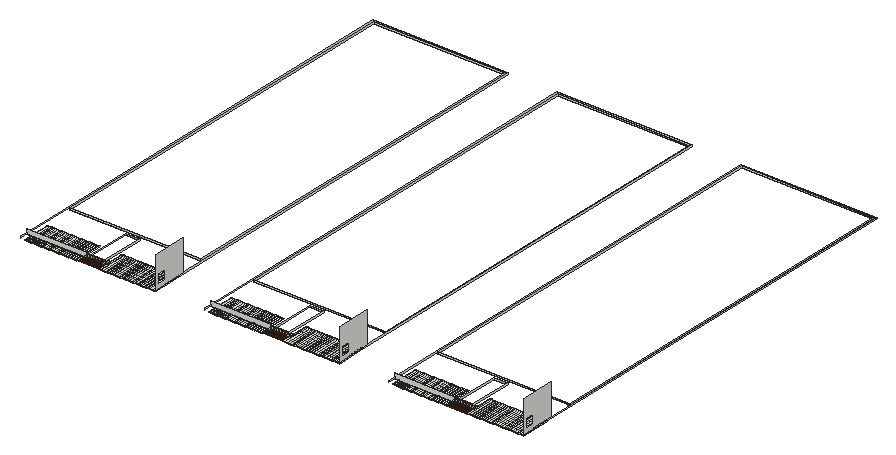
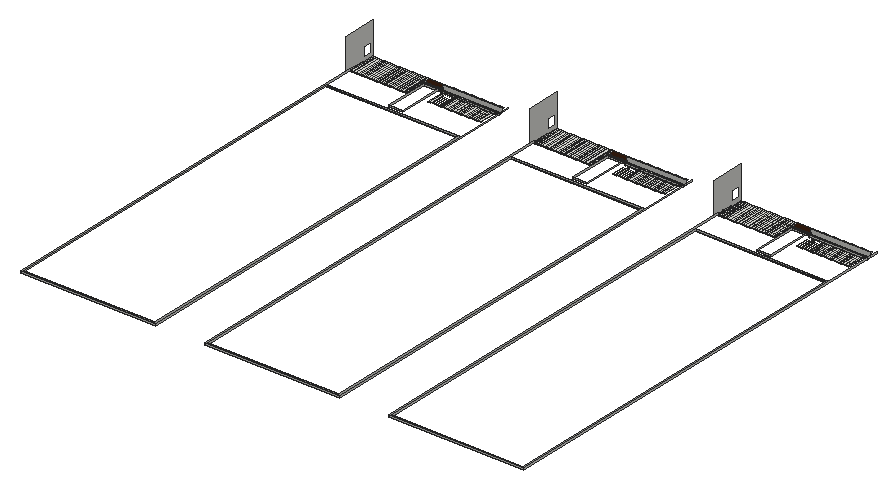
# SketchUp Ruby script. Lengths in inches.
U = 1.inch
M = Sketchup.active_model
def pt(a) = Geom::Point3d.new(a.map { |v| v * U })
def face(e, loops, mat)
  f = e.add_face(loops[0].map { |a| pt(a) })
  loops[1..].each { |l| e.add_face(l.map { |a| pt(a) }).erase! }
  f.material = f.back_material = mat if mat
  f
end
# faces: each face lists its corners as indices into pts; further lists are holes
def faces(e, pts, list, mat = nil) = list.each { |f| face(e, (f[0].is_a?(Array) ? f : [f]).map { |l| l.map { |i| pts[i] } }, mat) }
# xy, xz, yz: faces in a plane at the given z, y or x. An outline is a flat list of corners, or four numbers for a rectangle; further outlines are holes
def ring(l) = l.size == 4 ? [[l[0], l[1]], [l[2], l[1]], [l[2], l[3]], [l[0], l[3]]] : l.each_slice(2).to_a
def flat(e, list, mat, &to3) = list.each { |f| face(e, (f[0].is_a?(Array) ? f : [f]).map { |l| ring(l).map { |u, v| to3.(u, v) } }, mat) }
def xy(e, z, list, mat = nil) = flat(e, list, mat) { |x, y| [x, y, z] }
def xz(e, y, list, mat = nil) = flat(e, list, mat) { |x, z| [x, y, z] }
def yz(e, x, list, mat = nil) = flat(e, list, mat) { |y, z| [x, y, z] }
def lines(e, pts, list) = list.each { |a, b| e.add_line(pt(pts[a]), pt(pts[b])) }
# prism: a flat outline (further loops are holes) pulled along v
def prism(e, loops, v, mat = nil)
  f = face(e, loops, mat); d = Geom::Vector3d.new(v.map { |x| x * U })
  f.pushpull(f.normal.samedirection?(d) ? d.length : -d.length)
end
def box(e, o, s, mat = nil) = prism(e, [[o, [o[0] + s[0], o[1], o[2]], [o[0] + s[0], o[1] + s[1], o[2]], [o[0], o[1] + s[1], o[2]]]], [0, 0, s[2]], mat)
def at(x, y, z, deg = 0) = Geom::Transformation.translation(pt([x, y, z])) * Geom::Transformation.rotation(ORIGIN, Z_AXIS, deg.degrees)
def axes(o, x, y, z) = Geom::Transformation.new([*x, 0, *y, 0, *z, 0, *pt(o).to_a, 1])
def part(name) = M.definitions.add(name)
# library, detail: a bought-in or finely detailed component or shape, given as its bounding box
def library(name, o, s) = part(name).tap { |d| box(d.entities, o, s) }
def detail(e, o, s) = box(e.add_group.entities, o, s)
def put(e, d, t, mat = nil) = e.add_instance(d, t).tap { |i| i.material = mat if mat }
def group(e, t, mat = nil) = e.add_group.tap { |g| g.transformation = t; g.material = mat if mat }.entities
root = M.entities
M.materials.add("[Wood Veneer 01]").color = [51, 28, 15]
xy(root,505.1875,[[253.94,246.64,259.43,361.27],[987.51,246.64,993,361.27],[1721.07,246.64,1726.56,361.27]])
xy(root,505.3125,[[100.18,246.64,109.94,361.27],[109.94,246.64,115.43,361.27],[115.43,246.64,117.94,361.27],[117.94,246.64,123.43,361.27],[123.43,246.64,125.94,361.27],
  [125.94,246.64,131.43,361.27],[131.43,246.64,133.94,361.27],[133.94,246.64,139.43,361.27],[139.43,246.64,141.94,361.27],[141.94,246.64,147.43,361.27],
  [147.43,246.64,149.94,361.27],[149.94,246.64,155.43,361.27],[155.43,246.64,157.94,361.27],[157.94,246.64,163.43,361.27],[163.43,246.64,165.94,361.27],
  [165.94,246.64,171.43,361.27],[171.43,246.64,173.94,361.27],[173.94,246.64,179.43,361.27],[179.43,246.64,181.94,361.27],[181.94,246.64,187.43,361.27],
  [187.43,246.64,189.94,361.27],[189.94,246.64,195.43,361.27],[195.43,246.64,197.94,361.27],[197.94,246.64,203.43,361.27],[203.43,246.64,205.94,361.27],
  [205.94,246.64,211.43,361.27],[211.43,246.64,213.94,361.27],[213.94,246.64,219.43,361.27],[219.43,246.64,221.94,361.27],[221.94,246.64,227.43,361.27],
  [227.43,246.64,229.94,361.27],[229.94,246.64,235.43,361.27],[235.43,246.64,237.94,361.27],[237.94,246.64,243.43,361.27],[243.43,246.64,245.94,361.27],
  [245.94,246.64,251.43,361.27],[251.43,246.64,253.94,361.27],[259.43,246.64,261.94,361.27],[267.43,246.64,269.94,361.27],[275.43,246.64,277.94,361.27],
  [283.43,246.64,285.94,361.27],[291.43,246.64,293.94,361.27],[299.43,246.64,301.94,361.27],[307.43,246.64,309.94,361.27],[396.57,246.64,403.28,361.27],
  [403.28,246.64,405.07,361.27],[405.07,246.64,411.78,361.27],[411.78,246.64,413.57,361.27],[413.57,246.64,420.28,361.27],[420.28,246.64,422.07,361.27],
  [422.07,246.64,428.78,361.27],[428.78,246.64,430.57,361.27],[430.57,246.64,437.28,361.27],[437.28,246.64,439.07,361.27],[439.07,246.64,445.78,361.27],
  [445.78,246.64,447.57,361.27],[447.57,246.64,454.28,361.27],[454.28,246.64,456.07,361.27],[456.07,246.64,462.78,361.27],[462.78,246.64,464.57,361.27],
  [464.57,246.64,471.28,361.27],[471.28,246.64,473.07,361.27],[473.07,246.64,479.78,361.27],[479.78,246.64,481.57,361.27],[481.57,246.64,488.28,361.27],
  [488.28,246.64,490.07,361.27],[490.07,246.64,496.78,361.27],[496.78,246.64,498.57,361.27],[498.57,246.64,505.28,361.27],[505.28,246.64,507.07,361.27],
  [507.07,246.64,513.78,361.27],[513.78,246.64,515.57,361.27],[515.57,246.64,522.28,361.27],[522.28,246.64,524.07,361.27],[524.07,246.64,530.78,361.27],
  [530.78,246.64,532.57,361.27],[532.57,246.64,539.28,361.27],[539.28,246.64,541.07,361.27],[541.07,246.64,547.78,361.27],[547.78,246.64,549.57,361.27],
  [549.57,246.64,556.28,361.27],[556.28,246.64,558.07,361.27],[558.07,246.64,564.78,361.27],[564.78,246.64,566.57,361.27],[566.57,246.64,573.28,361.27],
  [573.28,246.64,575.07,361.27],[575.07,246.64,581.78,361.27],[581.78,246.64,583.57,361.27],[583.57,246.64,590.28,361.27],[590.28,246.64,592.07,361.27],
  [592.07,246.64,598.78,361.27],[598.78,246.64,600.57,361.27],[600.57,246.64,607.28,361.27],[607.28,246.64,609.07,361.27],[609.07,246.64,615.78,361.27],
  [615.78,246.64,617.57,361.27],[617.57,246.64,622,361.27],[833.74,246.64,843.51,361.27],[843.51,246.64,849,361.27],[849,246.64,851.51,361.27],
  [851.51,246.64,857,361.27],[857,246.64,859.51,361.27],[859.51,246.64,865,361.27],[865,246.64,867.51,361.27],[867.51,246.64,873,361.27],
  [873,246.64,875.51,361.27],[875.51,246.64,881,361.27],[881,246.64,883.51,361.27],[883.51,246.64,889,361.27],[889,246.64,891.51,361.27],
  [891.51,246.64,897,361.27],[897,246.64,899.51,361.27],[899.51,246.64,905,361.27],[905,246.64,907.51,361.27],[907.51,246.64,913,361.27],
  [913,246.64,915.51,361.27],[915.51,246.64,921,361.27],[921,246.64,923.51,361.27],[923.51,246.64,929,361.27],[929,246.64,931.51,361.27],
  [931.51,246.64,937,361.27],[937,246.64,939.51,361.27],[939.51,246.64,945,361.27],[945,246.64,947.51,361.27],[947.51,246.64,953,361.27],
  [953,246.64,955.51,361.27],[955.51,246.64,961,361.27],[961,246.64,963.51,361.27],[963.51,246.64,969,361.27],[969,246.64,971.51,361.27],
  [971.51,246.64,977,361.27],[977,246.64,979.51,361.27],[979.51,246.64,985,361.27],[985,246.64,987.51,361.27],[993,246.64,995.51,361.27],
  [1001,246.64,1003.51,361.27],[1009,246.64,1011.51,361.27],[1017,246.64,1019.51,361.27],[1025,246.64,1027.51,361.27],[1033,246.64,1035.51,361.27],
  [1041,246.64,1043.51,361.27],[1130.14,246.64,1136.84,361.27],[1136.84,246.64,1138.64,361.27],[1138.64,246.64,1145.34,361.27],[1145.34,246.64,1147.14,361.27],
  [1147.14,246.64,1153.84,361.27],[1153.84,246.64,1155.64,361.27],[1155.64,246.64,1162.34,361.27],[1162.34,246.64,1164.14,361.27],[1164.14,246.64,1170.84,361.27],
  [1170.84,246.64,1172.64,361.27],[1172.64,246.64,1179.34,361.27],[1179.34,246.64,1181.14,361.27],[1181.14,246.64,1187.84,361.27],[1187.84,246.64,1189.64,361.27],
  [1189.64,246.64,1196.34,361.27],[1196.34,246.64,1198.14,361.27],[1198.14,246.64,1204.84,361.27],[1204.84,246.64,1206.64,361.27],[1206.64,246.64,1213.34,361.27],
  [1213.34,246.64,1215.14,361.27],[1215.14,246.64,1221.84,361.27],[1221.84,246.64,1223.64,361.27],[1223.64,246.64,1230.34,361.27],[1230.34,246.64,1232.14,361.27],
  [1232.14,246.64,1238.84,361.27],[1238.84,246.64,1240.64,361.27],[1240.64,246.64,1247.34,361.27],[1247.34,246.64,1249.14,361.27],[1249.14,246.64,1255.84,361.27],
  [1255.84,246.64,1257.64,361.27],[1257.64,246.64,1264.34,361.27],[1264.34,246.64,1266.14,361.27],[1266.14,246.64,1272.84,361.27],[1272.84,246.64,1274.64,361.27],
  [1274.64,246.64,1281.34,361.27],[1281.34,246.64,1283.14,361.27],[1283.14,246.64,1289.84,361.27],[1289.84,246.64,1291.64,361.27],[1291.64,246.64,1298.34,361.27],
  [1298.34,246.64,1300.14,361.27],[1300.14,246.64,1306.84,361.27],[1306.84,246.64,1308.64,361.27],[1308.64,246.64,1315.34,361.27],[1315.34,246.64,1317.14,361.27],
  [1317.14,246.64,1323.84,361.27],[1323.84,246.64,1325.64,361.27],[1325.64,246.64,1332.34,361.27],[1332.34,246.64,1334.14,361.27],[1334.14,246.64,1340.84,361.27],
  [1340.84,246.64,1342.64,361.27],[1342.64,246.64,1349.34,361.27],[1349.34,246.64,1351.14,361.27],[1351.14,246.64,1355.5625,361.27],[1567.3,246.64,1577.07,361.27],
  [1577.07,246.64,1582.56,361.27],[1582.56,246.64,1585.07,361.27],[1585.07,246.64,1590.56,361.27],[1590.56,246.64,1593.07,361.27],[1593.07,246.64,1598.56,361.27],
  [1598.56,246.64,1601.07,361.27],[1601.07,246.64,1606.56,361.27],[1606.56,246.64,1609.07,361.27],[1609.07,246.64,1614.56,361.27],[1614.56,246.64,1617.07,361.27],
  [1617.07,246.64,1622.56,361.27],[1622.56,246.64,1625.07,361.27],[1625.07,246.64,1630.56,361.27],[1630.56,246.64,1633.07,361.27],[1633.07,246.64,1638.56,361.27],
  [1638.56,246.64,1641.07,361.27],[1641.07,246.64,1646.56,361.27],[1646.56,246.64,1649.07,361.27],[1649.07,246.64,1654.56,361.27],[1654.56,246.64,1657.07,361.27],
  [1657.07,246.64,1662.56,361.27],[1662.56,246.64,1665.07,361.27],[1665.07,246.64,1670.56,361.27],[1670.56,246.64,1673.07,361.27],[1673.07,246.64,1678.56,361.27],
  [1678.56,246.64,1681.07,361.27],[1681.07,246.64,1686.56,361.27],[1686.56,246.64,1689.07,361.27],[1689.07,246.64,1694.56,361.27],[1694.56,246.64,1697.07,361.27],
  [1697.07,246.64,1702.56,361.27],[1702.56,246.64,1705.07,361.27],[1705.07,246.64,1710.56,361.27],[1710.56,246.64,1713.07,361.27],[1713.07,246.64,1718.56,361.27],
  [1718.56,246.64,1721.07,361.27],[1726.56,246.64,1729.07,361.27],[1734.56,246.64,1737.07,361.27],[1742.56,246.64,1745.07,361.27],[1750.56,246.64,1753.07,361.27],
  [1758.56,246.64,1761.07,361.27],[1766.56,246.64,1769.07,361.27],[1774.56,246.64,1777.07,361.27],[1863.7,246.64,1870.4,361.27],[1870.4,246.64,1872.2,361.27],
  [1872.2,246.64,1878.9,361.27],[1878.9,246.64,1880.7,361.27],[1880.7,246.64,1887.4,361.27],[1887.4,246.64,1889.2,361.27],[1889.2,246.64,1895.9,361.27],
  [1895.9,246.64,1897.7,361.27],[1897.7,246.64,1904.4,361.27],[1904.4,246.64,1906.2,361.27],[1906.2,246.64,1912.9,361.27],[1912.9,246.64,1914.7,361.27],
  [1914.7,246.64,1921.4,361.27],[1921.4,246.64,1923.2,361.27],[1923.2,246.64,1929.9,361.27],[1929.9,246.64,1931.7,361.27],[1931.7,246.64,1938.4,361.27],
  [1938.4,246.64,1940.2,361.27],[1940.2,246.64,1946.9,361.27],[1946.9,246.64,1948.7,361.27],[1948.7,246.64,1955.4,361.27],[1955.4,246.64,1957.2,361.27],
  [1957.2,246.64,1963.9,361.27],[1963.9,246.64,1965.7,361.27],[1965.7,246.64,1972.4,361.27],[1972.4,246.64,1974.2,361.27],[1974.2,246.64,1980.9,361.27],
  [1980.9,246.64,1982.7,361.27],[1982.7,246.64,1989.4,361.27],[1989.4,246.64,1991.2,361.27],[1991.2,246.64,1997.9,361.27],[1997.9,246.64,1999.7,361.27],
  [1999.7,246.64,2006.4,361.27],[2006.4,246.64,2008.2,361.27],[2008.2,246.64,2014.9,361.27],[2014.9,246.64,2016.7,361.27],[2016.7,246.64,2023.4,361.27],
  [2023.4,246.64,2025.2,361.27],[2025.2,246.64,2031.9,361.27],[2031.9,246.64,2033.7,361.27],[2033.7,246.64,2040.4,361.27],[2040.4,246.64,2042.2,361.27],
  [2042.2,246.64,2048.9,361.27],[2048.9,246.64,2050.7,361.27],[2050.7,246.64,2057.4,361.27],[2057.4,246.64,2059.2,361.27],[2059.2,246.64,2065.9,361.27],
  [2065.9,246.64,2067.7,361.27],[2067.7,246.64,2074.4,361.27],[2074.4,246.64,2076.2,361.27],[2076.2,246.64,2082.9,361.27],[2082.9,246.64,2084.7,361.27],
  [2084.7,246.64,2089.125,361.27]])
xy(root,505.3125,[[315.43,246.64,396.57,286.21],[1049,246.64,1130.14,286.21],[1782.56,246.64,1863.7,286.21]],"[Wood Veneer 01]")
xy(root,506.6875,[[106.73,254.22,113.67,256.84],[119.31,254.22,126.24,256.84],[132.68,254.22,139.62,256.84],[146.56,254.22,153.49,256.84],[840.29,254.22,847.23,256.84],
  [852.87,254.22,859.81,256.84],[866.24,254.22,873.18,256.84],[880.12,254.22,887.06,256.84],[1573.86,254.22,1580.79,256.84],[1586.43,254.22,1593.37,256.84],
  [1599.81,254.22,1606.74,256.84],[1613.68,254.22,1620.62,256.84],[106.73,256.84,113.67,263.78],[119.31,256.84,126.24,263.78],[132.68,256.84,139.62,263.78],
  [146.56,256.84,153.49,263.78],[840.29,256.84,847.23,263.78],[852.87,256.84,859.81,263.78],[866.24,256.84,873.18,263.78],[880.12,256.84,887.06,263.78],
  [1573.86,256.84,1580.79,263.78],[1586.43,256.84,1593.37,263.78],[1599.81,256.84,1606.74,263.78],[1613.68,256.84,1620.62,263.78],[90.36,483.79,614.76,488.08],
  [823.93,483.79,1348.32,488.08],[1557.49,483.79,2081.89,488.08]])
xy(root,506.8125,[[83.125,277.39,100.18,293.46],[100.18,277.39,100.18,293.46,315.43,293.46,315.43,286.21,318.81,286.21,318.81,277.39],[816.6875,277.39,833.74,293.46],[833.74,277.39,833.74,293.46,1049,293.46,1049,286.21,1052.37,286.21,1052.37,277.39],[1550.25,277.39,1567.3,293.46],
  [1567.3,277.39,1567.3,293.46,1782.56,293.46,1782.56,286.21,1785.93,286.21,1785.93,277.39]])
xz(root,246.64,[[259.43,505.1875,261.94,505.19,261.94,505.3125,259.43,505.3125],[993,505.1875,995.51,505.19,995.51,505.3125,993,505.3125],[1726.56,505.1875,1729.07,505.19,1729.07,505.3125,1726.56,505.3125],[267.43,505.21,269.94,505.3125],[1001,505.21,1003.51,505.3125],
  [1734.56,505.21,1737.07,505.3125],[275.43,505.22,277.94,505.23,277.94,505.3125,275.43,505.3125],[1009,505.22,1011.51,505.23,1011.51,505.3125,1009,505.3125],[1742.56,505.22,1745.07,505.23,1745.07,505.3125,1742.56,505.3125],[283.43,505.24,285.94,505.25,285.94,505.3125,283.43,505.3125],
  [1017,505.24,1019.51,505.25,1019.51,505.3125,1017,505.3125],[1750.56,505.24,1753.07,505.25,1753.07,505.3125,1750.56,505.3125],[291.43,505.26,293.94,505.3125],[1025,505.26,1027.51,505.3125],[1758.56,505.26,1761.07,505.3125],
  [299.43,505.28,301.94,505.3125],[1033,505.28,1035.51,505.3125],[1766.56,505.28,1769.07,505.3125],[307.43,505.29,309.94,505.3,309.94,505.3125,307.43,505.3125],[1041,505.29,1043.51,505.3,1043.51,505.3125,1041,505.3125],
  [1774.56,505.29,1777.07,505.3,1777.07,505.3125,1774.56,505.3125]])
xz(root,277.39,[[83.125,506.8125,318.81,524.9375],[816.6875,506.8125,1052.37,524.9375],[1550.25,506.8125,1785.93,524.9375]])
xz(root,286.21,[[315.43,505.3125,318.81,506.8125],[318.81,505.3125,322.23,506.8125],[322.23,505.3125,324.81,506.8125],[324.81,505.3125,328.23,506.8125],[328.23,505.3125,330.81,506.8125],
  [330.81,505.3125,334.23,506.8125],[334.23,505.3125,336.81,506.8125],[336.81,505.3125,340.23,506.8125],[340.23,505.3125,342.81,506.8125],[342.81,505.3125,346.23,506.8125],
  [346.23,505.3125,348.81,506.8125],[348.81,505.3125,352.23,506.8125],[352.23,505.3125,354.81,506.8125],[354.81,505.3125,358.23,506.8125],[358.23,505.3125,360.81,506.8125],
  [360.81,505.3125,364.23,506.8125],[364.23,505.3125,366.81,506.8125],[366.81,505.3125,370.23,506.8125],[370.23,505.3125,372.81,506.8125],[372.81,505.3125,376.23,506.8125],
  [376.23,505.3125,378.81,506.8125],[378.81,505.3125,382.23,506.8125],[382.23,505.3125,384.81,506.8125],[384.81,505.3125,388.23,506.8125],[388.23,505.3125,390.12,506.8125],
  [390.12,505.3125,393.55,506.8125],[393.55,505.3125,393.95,506.8125],[393.95,505.3125,396.57,506.8125],[1049,505.3125,1052.37,506.8125],[1052.37,505.3125,1055.8,506.8125],
  [1055.8,505.3125,1058.37,506.8125],[1058.37,505.3125,1061.8,506.8125],[1061.8,505.3125,1064.37,506.8125],[1064.37,505.3125,1067.8,506.8125],[1067.8,505.3125,1070.37,506.8125],
  [1070.37,505.3125,1073.8,506.8125],[1073.8,505.3125,1076.37,506.8125],[1076.37,505.3125,1079.8,506.8125],[1079.8,505.3125,1082.37,506.8125],[1082.37,505.3125,1085.8,506.8125],
  [1085.8,505.3125,1088.37,506.8125],[1088.37,505.3125,1091.8,506.8125],[1091.8,505.3125,1094.37,506.8125],[1094.37,505.3125,1097.8,506.8125],[1097.8,505.3125,1100.37,506.8125],
  [1100.37,505.3125,1103.8,506.8125],[1103.8,505.3125,1106.37,506.8125],[1106.37,505.3125,1109.8,506.8125],[1109.8,505.3125,1112.37,506.8125],[1112.37,505.3125,1115.8,506.8125],
  [1115.8,505.3125,1118.37,506.8125],[1118.37,505.3125,1121.8,506.8125],[1121.8,505.3125,1123.68,506.8125],[1123.68,505.3125,1127.11,506.8125],[1127.11,505.3125,1127.51,506.8125],
  [1127.51,505.3125,1130.14,506.8125],[1782.56,505.3125,1785.93,506.8125],[1785.93,505.3125,1789.36,506.8125],[1789.36,505.3125,1791.93,506.8125],[1791.93,505.3125,1795.36,506.8125],
  [1795.36,505.3125,1797.93,506.8125],[1797.93,505.3125,1801.36,506.8125],[1801.36,505.3125,1803.93,506.8125],[1803.93,505.3125,1807.36,506.8125],[1807.36,505.3125,1809.93,506.8125],
  [1809.93,505.3125,1813.36,506.8125],[1813.36,505.3125,1815.93,506.8125],[1815.93,505.3125,1819.36,506.8125],[1819.36,505.3125,1821.93,506.8125],[1821.93,505.3125,1825.36,506.8125],
  [1825.36,505.3125,1827.93,506.8125],[1827.93,505.3125,1831.36,506.8125],[1831.36,505.3125,1833.93,506.8125],[1833.93,505.3125,1837.36,506.8125],[1837.36,505.3125,1839.93,506.8125],
  [1839.93,505.3125,1843.36,506.8125],[1843.36,505.3125,1845.93,506.8125],[1845.93,505.3125,1849.36,506.8125],[1849.36,505.3125,1851.93,506.8125],[1851.93,505.3125,1855.36,506.8125],
  [1855.36,505.3125,1857.25,506.8125],[1857.25,505.3125,1860.67,506.8125],[1860.67,505.3125,1861.07,506.8125],[1861.07,505.3125,1863.7,506.8125],[315.43,506.8125,318.81,512.6875],
  [318.81,506.8125,322.23,512.6875],[322.23,506.8125,324.81,512.6875],[324.81,506.8125,328.23,512.6875],[328.23,506.8125,330.81,512.6875],[330.81,506.8125,334.23,512.6875],
  [334.23,506.8125,336.81,512.6875],[336.81,506.8125,340.23,512.6875],[340.23,506.8125,342.81,512.6875],[342.81,506.8125,346.23,512.6875],[346.23,506.8125,348.81,512.6875],
  [348.81,506.8125,352.23,512.6875],[352.23,506.8125,354.81,512.6875],[354.81,506.8125,358.23,512.6875],[358.23,506.8125,360.81,512.6875],[360.81,506.8125,364.23,512.6875],
  [364.23,506.8125,366.81,512.6875],[366.81,506.8125,370.23,512.6875],[370.23,506.8125,372.81,512.6875],[372.81,506.8125,376.23,512.6875],[376.23,506.8125,378.81,512.6875],
  [378.81,506.8125,382.23,512.6875],[382.23,506.8125,384.81,512.6875],[384.81,506.8125,388.23,512.6875],[388.23,506.8125,390.12,512.6875],[390.12,506.8125,393.55,512.6875],
  [393.55,506.8125,393.95,512.6875],[393.95,506.8125,396.57,512.6875],[1049,506.8125,1052.37,512.6875],[1052.37,506.8125,1055.8,512.6875],[1055.8,506.8125,1058.37,512.6875],
  [1058.37,506.8125,1061.8,512.6875],[1061.8,506.8125,1064.37,512.6875],[1064.37,506.8125,1067.8,512.6875],[1067.8,506.8125,1070.37,512.6875],[1070.37,506.8125,1073.8,512.6875],
  [1073.8,506.8125,1076.37,512.6875],[1076.37,506.8125,1079.8,512.6875],[1079.8,506.8125,1082.37,512.6875],[1082.37,506.8125,1085.8,512.6875],[1085.8,506.8125,1088.37,512.6875],
  [1088.37,506.8125,1091.8,512.6875],[1091.8,506.8125,1094.37,512.6875],[1094.37,506.8125,1097.8,512.6875],[1097.8,506.8125,1100.37,512.6875],[1100.37,506.8125,1103.8,512.6875],
  [1103.8,506.8125,1106.37,512.6875],[1106.37,506.8125,1109.8,512.6875],[1109.8,506.8125,1112.37,512.6875],[1112.37,506.8125,1115.8,512.6875],[1115.8,506.8125,1118.37,512.6875],
  [1118.37,506.8125,1121.8,512.6875],[1121.8,506.8125,1123.68,512.6875],[1123.68,506.8125,1127.11,512.6875],[1127.11,506.8125,1127.51,512.6875],[1127.51,506.8125,1130.14,512.6875],
  [1782.56,506.8125,1785.93,512.6875],[1785.93,506.8125,1789.36,512.6875],[1789.36,506.8125,1791.93,512.6875],[1791.93,506.8125,1795.36,512.6875],[1795.36,506.8125,1797.93,512.6875],
  [1797.93,506.8125,1801.36,512.6875],[1801.36,506.8125,1803.93,512.6875],[1803.93,506.8125,1807.36,512.6875],[1807.36,506.8125,1809.93,512.6875],[1809.93,506.8125,1813.36,512.6875],
  [1813.36,506.8125,1815.93,512.6875],[1815.93,506.8125,1819.36,512.6875],[1819.36,506.8125,1821.93,512.6875],[1821.93,506.8125,1825.36,512.6875],[1825.36,506.8125,1827.93,512.6875],
  [1827.93,506.8125,1831.36,512.6875],[1831.36,506.8125,1833.93,512.6875],[1833.93,506.8125,1837.36,512.6875],[1837.36,506.8125,1839.93,512.6875],[1839.93,506.8125,1843.36,512.6875],
  [1843.36,506.8125,1845.93,512.6875],[1845.93,506.8125,1849.36,512.6875],[1849.36,506.8125,1851.93,512.6875],[1851.93,506.8125,1855.36,512.6875],[1855.36,506.8125,1857.25,512.6875],
  [1857.25,506.8125,1860.67,512.6875],[1860.67,506.8125,1861.07,512.6875],[1861.07,506.8125,1863.7,512.6875]])
xz(root,293.45,[[328.03,506.6875,382.74,512.6875],[1061.59,506.6875,1116.3,512.6875],[1795.15,506.6875,1849.87,512.6875]])
xz(root,293.46,[[83.125,506.8125,90.36,512.6875],[90.36,506.8125,315.43,512.6875],[816.6875,506.8125,823.93,512.6875],[823.93,506.8125,1049,512.6875],[1550.25,506.8125,1557.49,512.6875],
  [1557.49,506.8125,1782.56,512.6875]])
xz(root,361.27,[[396.57,505.3125,614.76,506.8125],[614.76,505.3125,622,506.8125],[1130.14,505.3125,1348.32,506.8125],[1348.32,505.3125,1355.5625,506.8125],[1863.7,505.3125,2081.89,506.8125],
  [2081.89,505.3125,2089.125,506.8125]])
xz(root,465.02,[[328.03,506.6875,382.74,512.6875],[1061.59,506.6875,1116.3,512.6875],[1795.15,506.6875,1849.87,512.6875]])
xz(root,483.79,[[90.36,506.6875,614.76,512.6875],[823.93,506.6875,1348.32,512.6875],[1557.49,506.6875,2081.89,512.6875]])
xz(root,1996.66,[[90.36,506.6875,614.76,512.6875],[823.93,506.6875,1348.32,512.6875],[1557.49,506.6875,2081.89,512.6875]])
xz(root,2003.89,[[83.125,506.6875,622,512.6875],[816.6875,506.6875,1355.5625,512.6875],[1550.25,506.6875,2089.125,512.6875]])
yz(root,83.125,[[246.64,506.6875,246.64,512.6875,277.39,512.6875,277.39,506.8125,293.46,506.8125,293.46,506.6875],[293.46,506.6875,2003.89,512.6875],[277.39,506.8125,293.46,512.6875]])
yz(root,90.36,[[483.79,506.6875,1996.66,512.6875]])
yz(root,100.18,[[246.64,505.3125,293.46,506.8125],[293.46,505.3125,361.27,506.8125]])
yz(root,253.94,[[246.64,505.1875,361.27,505.3125]])
yz(root,259.43,[[246.64,505.1875,286.21,505.3125],[286.21,505.1875,293.45,505.3125],[293.45,505.1875,293.46,505.3125],[293.46,505.1875,361.27,505.3125]])
yz(root,315.43,[[286.21,506.8125,293.45,512.6875],[293.45,506.8125,293.46,512.6875]])
yz(root,318.81,[[271.96,506.6875,271.96,512.6875,277.39,512.6875,277.39,506.8125,286.21,506.8125,286.21,506.6875],[277.39,506.8125,286.21,512.6875]])
yz(root,324.81,[[282.52,506.6875,286.21,512.6875]])
yz(root,328.03,[[293.45,506.6875,465.02,512.6875]])
yz(root,330.81,[[282.52,506.6875,286.21,512.6875]])
yz(root,336.81,[[282.52,506.6875,286.21,512.6875]])
yz(root,342.81,[[282.52,506.6875,286.21,512.6875]])
yz(root,348.81,[[283.46,506.6875,286.21,512.6875]])
yz(root,354.81,[[283.46,506.6875,286.21,512.6875]])
yz(root,360.81,[[283.46,506.6875,286.21,512.6875]])
yz(root,366.81,[[283.46,506.6875,286.21,512.6875]])
yz(root,372.81,[[283.46,506.6875,286.21,512.6875]])
yz(root,378.81,[[283.46,506.6875,286.21,512.6875]])
yz(root,382.74,[[293.45,506.6875,465.02,512.6875]])
yz(root,384.81,[[283.46,506.6875,286.21,512.6875]])
yz(root,390.12,[[272.89,506.6875,286.21,512.6875]])
yz(root,396.57,[[286.21,505.3125,293.45,506.8125],[293.45,505.3125,361.27,506.8125],[286.21,506.8125,293.45,512.6875]])
yz(root,614.76,[[483.79,506.6875,1996.66,512.6875]])
yz(root,622,[[246.64,505.3125,293.45,506.8125],[293.45,505.3125,361.27,506.8125],[361.27,506.6875,2003.89,512.6875],[246.64,506.8125,293.45,506.8125,293.45,524.9375,258.35,524.9375,258.35,560.9375,293.45,560.9375,293.45,512.6875,381.35,512.6875,381.35,636.53,246.64,636.53],[293.45,506.8125,361.27,512.6875]])
yz(root,816.6875,[[246.64,506.6875,246.64,512.6875,277.39,512.6875,277.39,506.8125,293.46,506.8125,293.46,506.6875],[293.46,506.6875,2003.89,512.6875],[277.39,506.8125,293.46,512.6875]])
yz(root,823.93,[[483.79,506.6875,1996.66,512.6875]])
yz(root,833.74,[[246.64,505.3125,293.46,506.8125],[293.46,505.3125,361.27,506.8125]])
yz(root,987.51,[[246.64,505.1875,361.27,505.3125]])
yz(root,993,[[246.64,505.1875,286.21,505.3125],[286.21,505.1875,293.45,505.3125],[293.45,505.1875,293.46,505.3125],[293.46,505.1875,361.27,505.3125]])
yz(root,1049,[[286.21,506.8125,293.45,512.6875],[293.45,506.8125,293.46,512.6875]])
yz(root,1052.37,[[271.96,506.6875,271.96,512.6875,277.39,512.6875,277.39,506.8125,286.21,506.8125,286.21,506.6875],[277.39,506.8125,286.21,512.6875]])
yz(root,1058.37,[[282.52,506.6875,286.21,512.6875]])
yz(root,1061.59,[[293.45,506.6875,465.02,512.6875]])
yz(root,1064.37,[[282.52,506.6875,286.21,512.6875]])
yz(root,1070.37,[[282.52,506.6875,286.21,512.6875]])
yz(root,1076.37,[[282.52,506.6875,286.21,512.6875]])
yz(root,1082.37,[[283.46,506.6875,286.21,512.6875]])
yz(root,1088.37,[[283.46,506.6875,286.21,512.6875]])
yz(root,1094.37,[[283.46,506.6875,286.21,512.6875]])
yz(root,1100.37,[[283.46,506.6875,286.21,512.6875]])
yz(root,1106.37,[[283.46,506.6875,286.21,512.6875]])
yz(root,1112.37,[[283.46,506.6875,286.21,512.6875]])
yz(root,1116.3,[[293.45,506.6875,465.02,512.6875]])
yz(root,1118.37,[[283.46,506.6875,286.21,512.6875]])
yz(root,1123.68,[[272.89,506.6875,286.21,512.6875]])
yz(root,1130.14,[[286.21,505.3125,293.45,506.8125],[293.45,505.3125,361.27,506.8125],[286.21,506.8125,293.45,512.6875]])
yz(root,1348.32,[[483.79,506.6875,1996.66,512.6875]])
yz(root,1355.5625,[[246.64,505.3125,293.45,506.8125],[293.45,505.3125,361.27,506.8125],[361.27,506.6875,2003.89,512.6875],[246.64,506.8125,293.45,506.8125,293.45,524.9375,258.35,524.9375,258.35,560.9375,293.45,560.9375,293.45,512.6875,381.35,512.6875,381.35,636.53,246.64,636.53],[293.45,506.8125,361.27,512.6875]])
yz(root,1550.25,[[246.64,506.6875,246.64,512.6875,277.39,512.6875,277.39,506.8125,293.46,506.8125,293.46,506.6875],[293.46,506.6875,2003.89,512.6875],[277.39,506.8125,293.46,512.6875]])
yz(root,1557.49,[[483.79,506.6875,1996.66,512.6875]])
yz(root,1567.3,[[246.64,505.3125,293.46,506.8125],[293.46,505.3125,361.27,506.8125]])
yz(root,1721.07,[[246.64,505.1875,361.27,505.3125]])
yz(root,1726.56,[[246.64,505.1875,286.21,505.3125],[286.21,505.1875,293.45,505.3125],[293.45,505.1875,293.46,505.3125],[293.46,505.1875,361.27,505.3125]])
yz(root,1782.56,[[286.21,506.8125,293.45,512.6875],[293.45,506.8125,293.46,512.6875]])
yz(root,1785.93,[[271.96,506.6875,271.96,512.6875,277.39,512.6875,277.39,506.8125,286.21,506.8125,286.21,506.6875],[277.39,506.8125,286.21,512.6875]])
yz(root,1791.93,[[282.52,506.6875,286.21,512.6875]])
yz(root,1795.15,[[293.45,506.6875,465.02,512.6875]])
yz(root,1797.93,[[282.52,506.6875,286.21,512.6875]])
yz(root,1803.93,[[282.52,506.6875,286.21,512.6875]])
yz(root,1809.93,[[282.52,506.6875,286.21,512.6875]])
yz(root,1815.93,[[283.46,506.6875,286.21,512.6875]])
yz(root,1821.93,[[283.46,506.6875,286.21,512.6875]])
yz(root,1827.93,[[283.46,506.6875,286.21,512.6875]])
yz(root,1833.93,[[283.46,506.6875,286.21,512.6875]])
yz(root,1839.93,[[283.46,506.6875,286.21,512.6875]])
yz(root,1845.93,[[283.46,506.6875,286.21,512.6875]])
yz(root,1849.87,[[293.45,506.6875,465.02,512.6875]])
yz(root,1851.93,[[283.46,506.6875,286.21,512.6875]])
yz(root,1857.25,[[272.89,506.6875,286.21,512.6875]])
yz(root,1863.7,[[286.21,505.3125,293.45,506.8125],[293.45,505.3125,361.27,506.8125],[286.21,506.8125,293.45,512.6875]])
yz(root,2081.89,[[483.79,506.6875,1996.66,512.6875]])
yz(root,2089.125,[[246.64,505.3125,293.45,506.8125],[293.45,505.3125,361.27,506.8125],[361.27,506.6875,2003.89,512.6875],[246.64,506.8125,293.45,506.8125,293.45,524.9375,258.35,524.9375,258.35,560.9375,293.45,560.9375,293.45,512.6875,381.35,512.6875,381.35,636.53,246.64,636.53],[293.45,506.8125,361.27,512.6875]])
p = [[823.93,293.46,506.6875],[833.74,293.46,506.6875],[823.93,293.46,506.8125],[1557.49,293.46,506.6875],[1567.3,293.46,506.6875],[1557.49,293.46,506.8125],
  [90.36,293.46,506.6875],[100.18,293.46,506.6875],[90.36,293.46,506.8125]]
lines(root,p,[[0,1],[0,2],[3,4],[3,5],[6,7],[6,8]])
